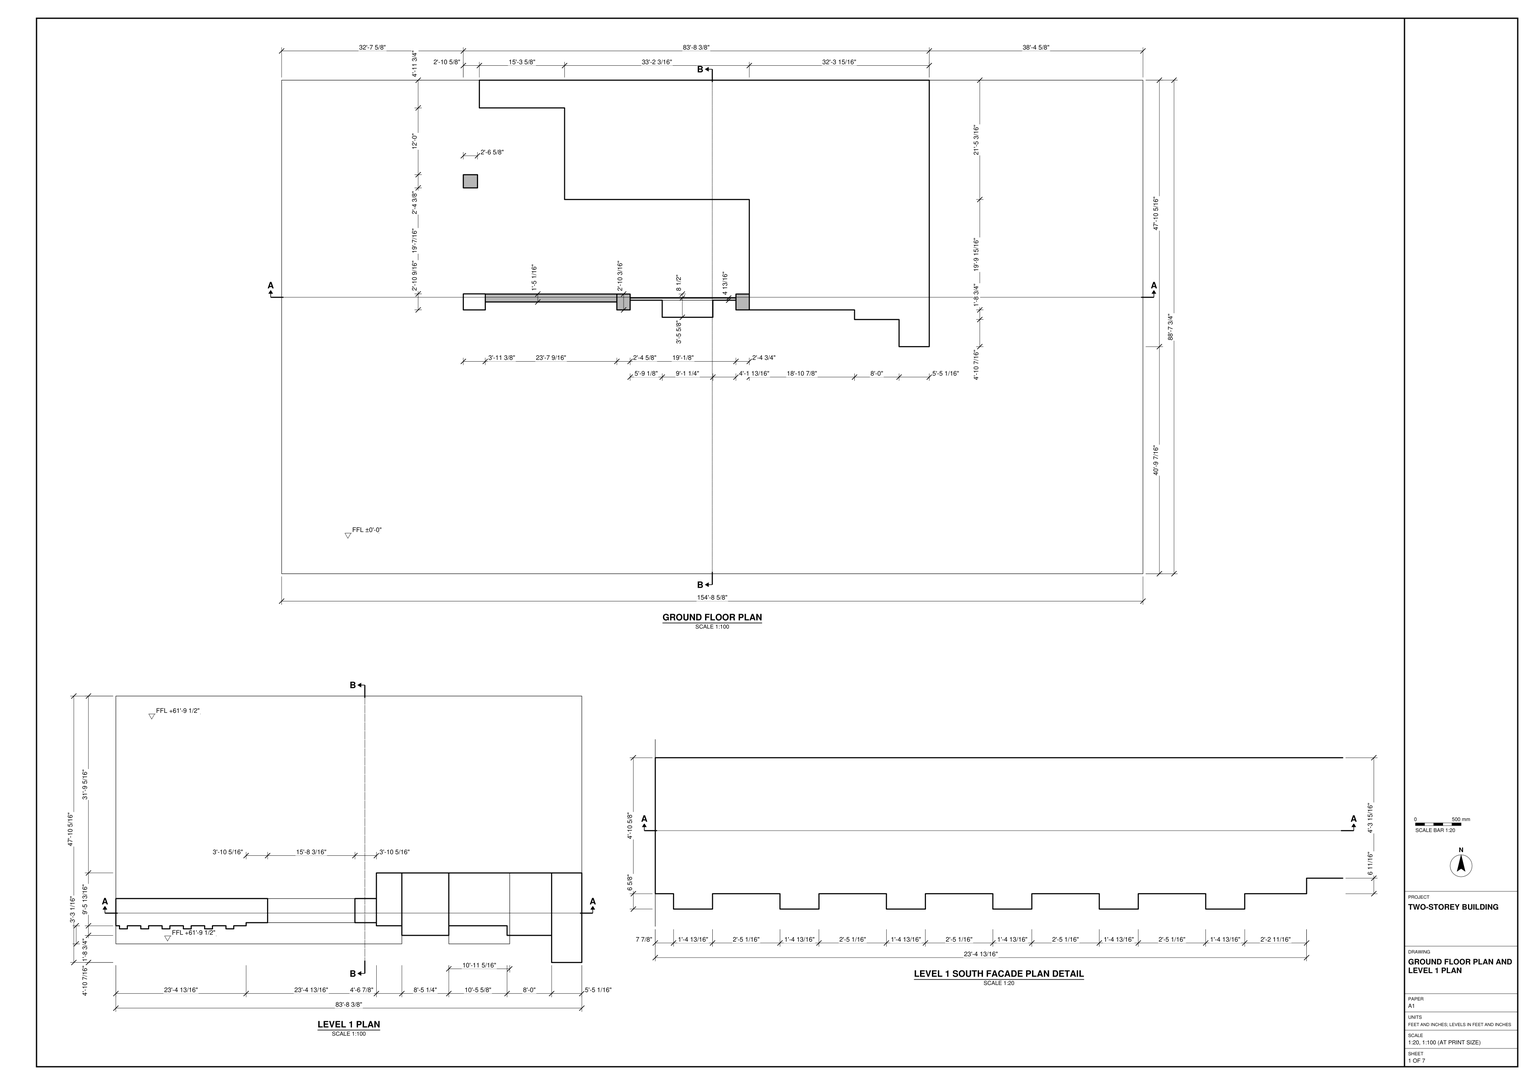
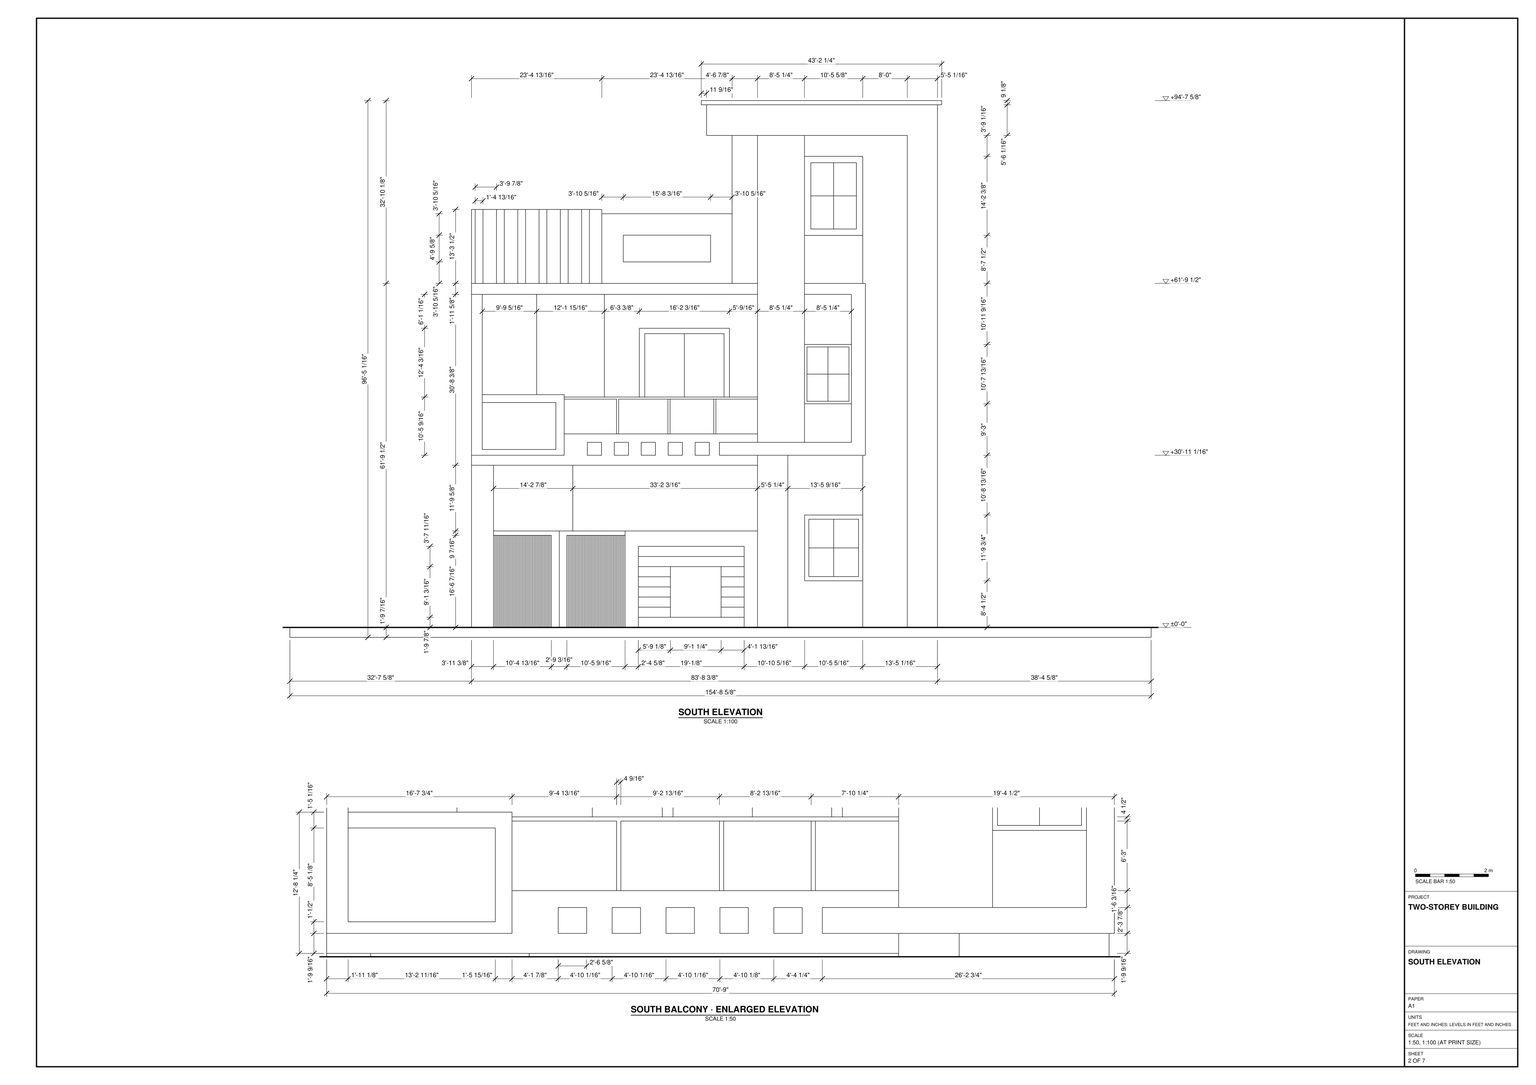
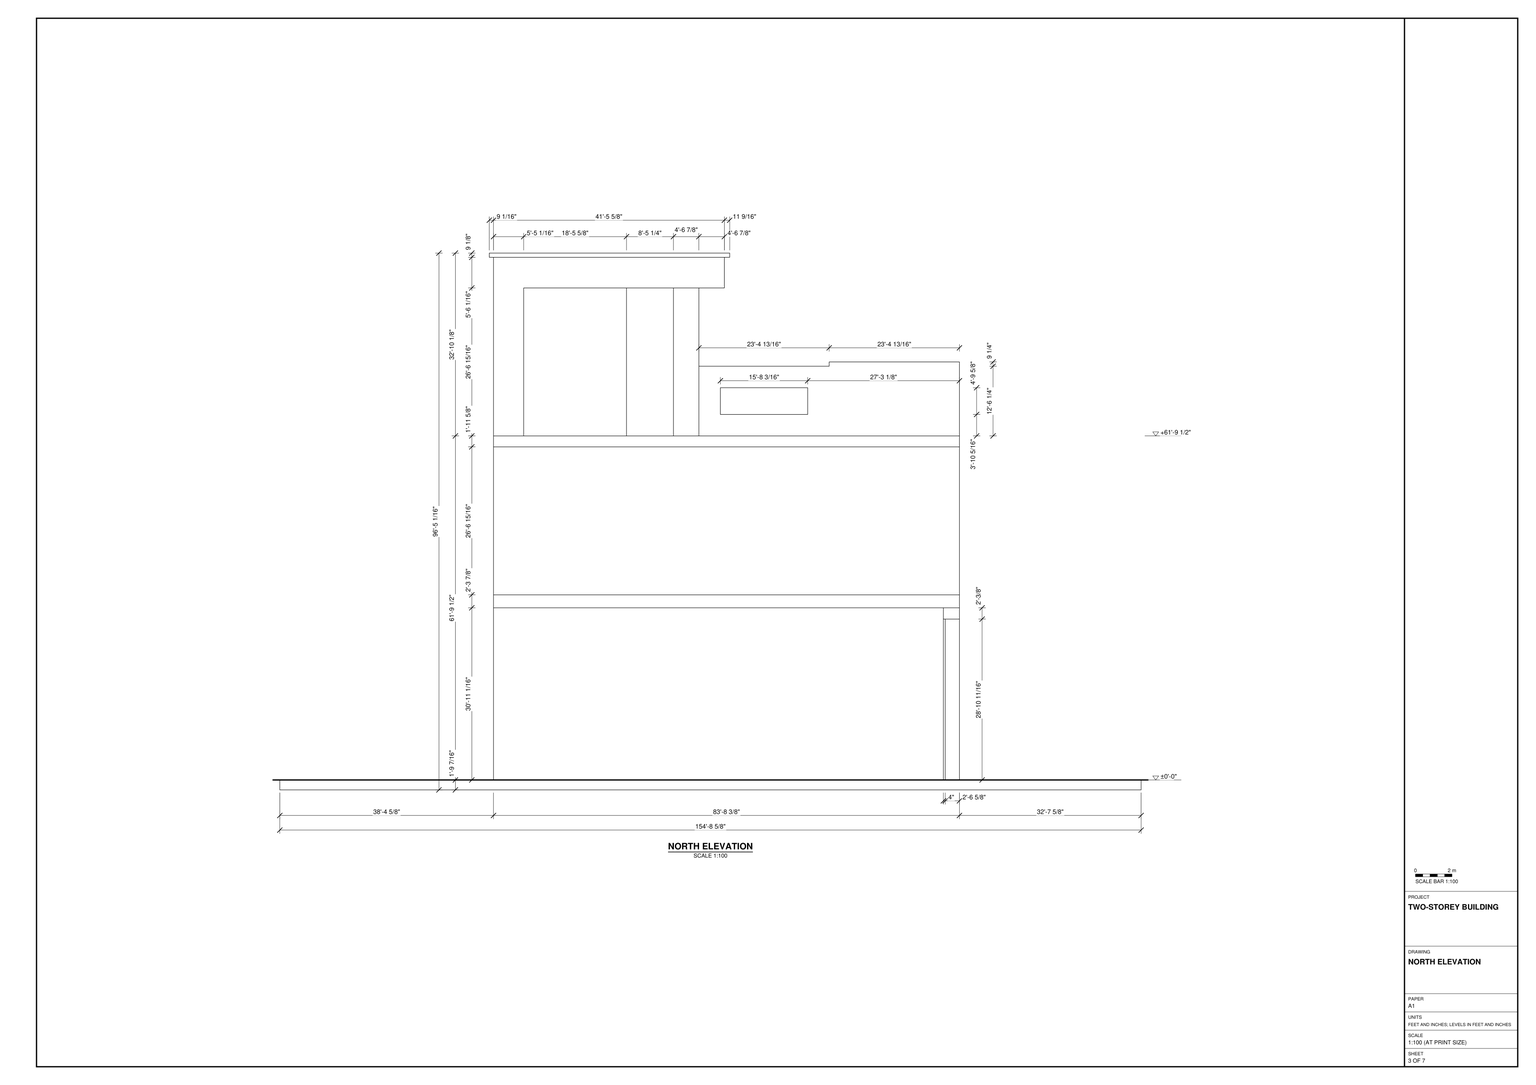
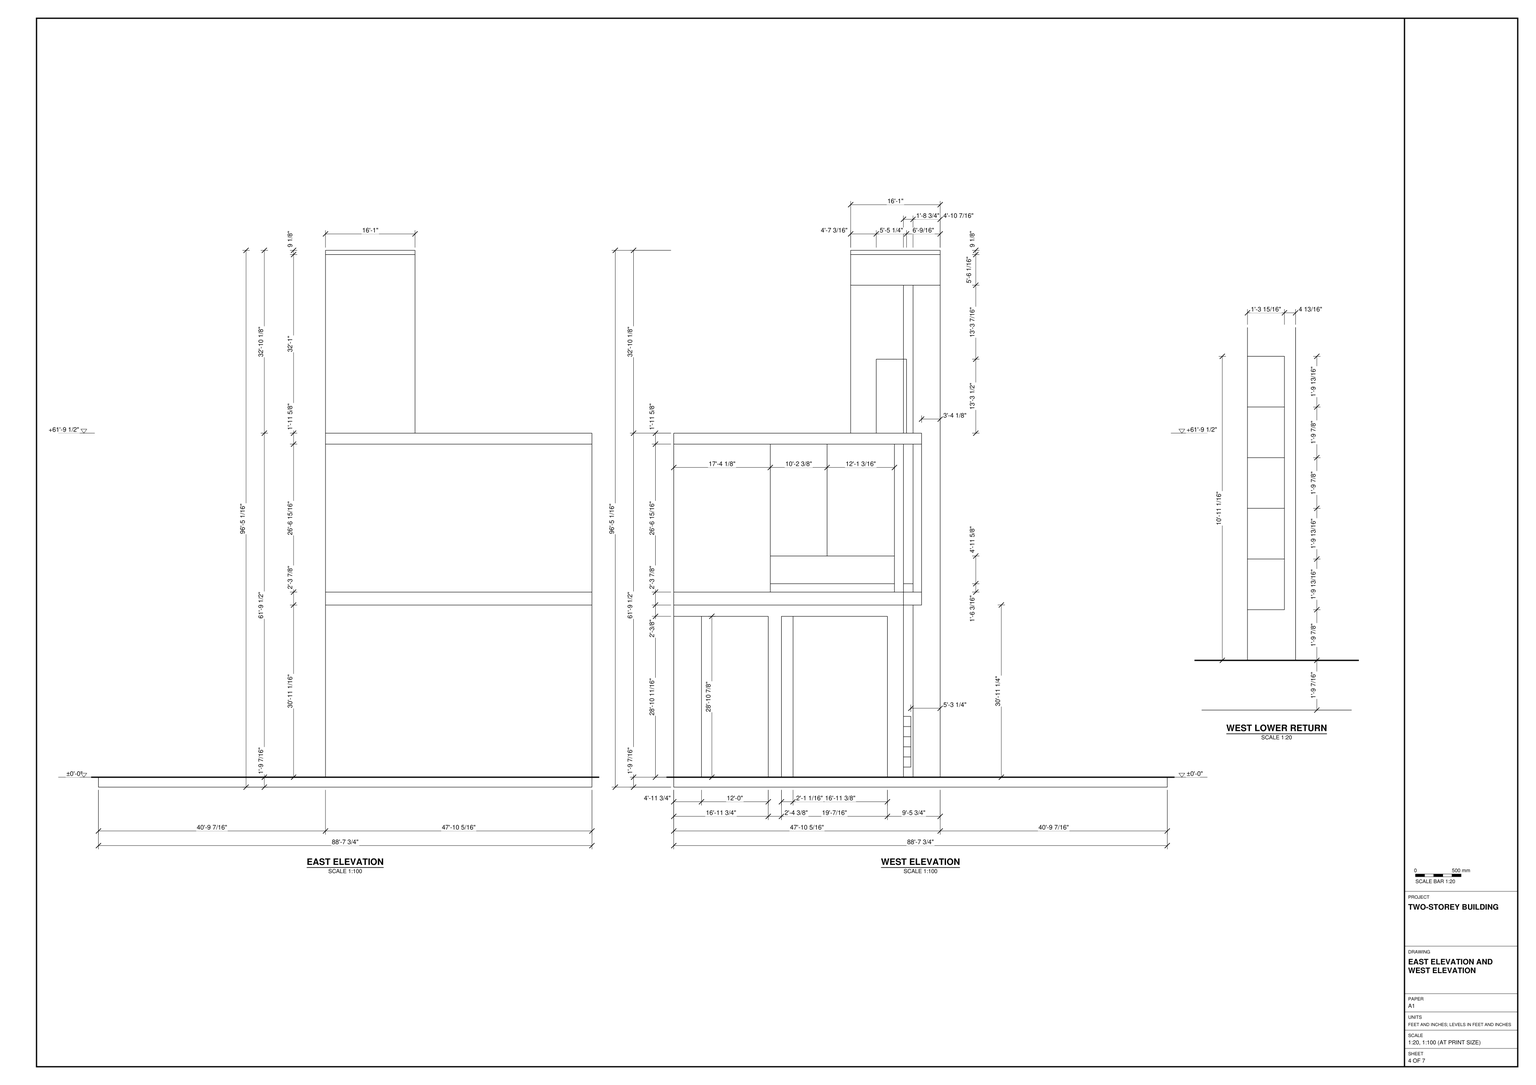
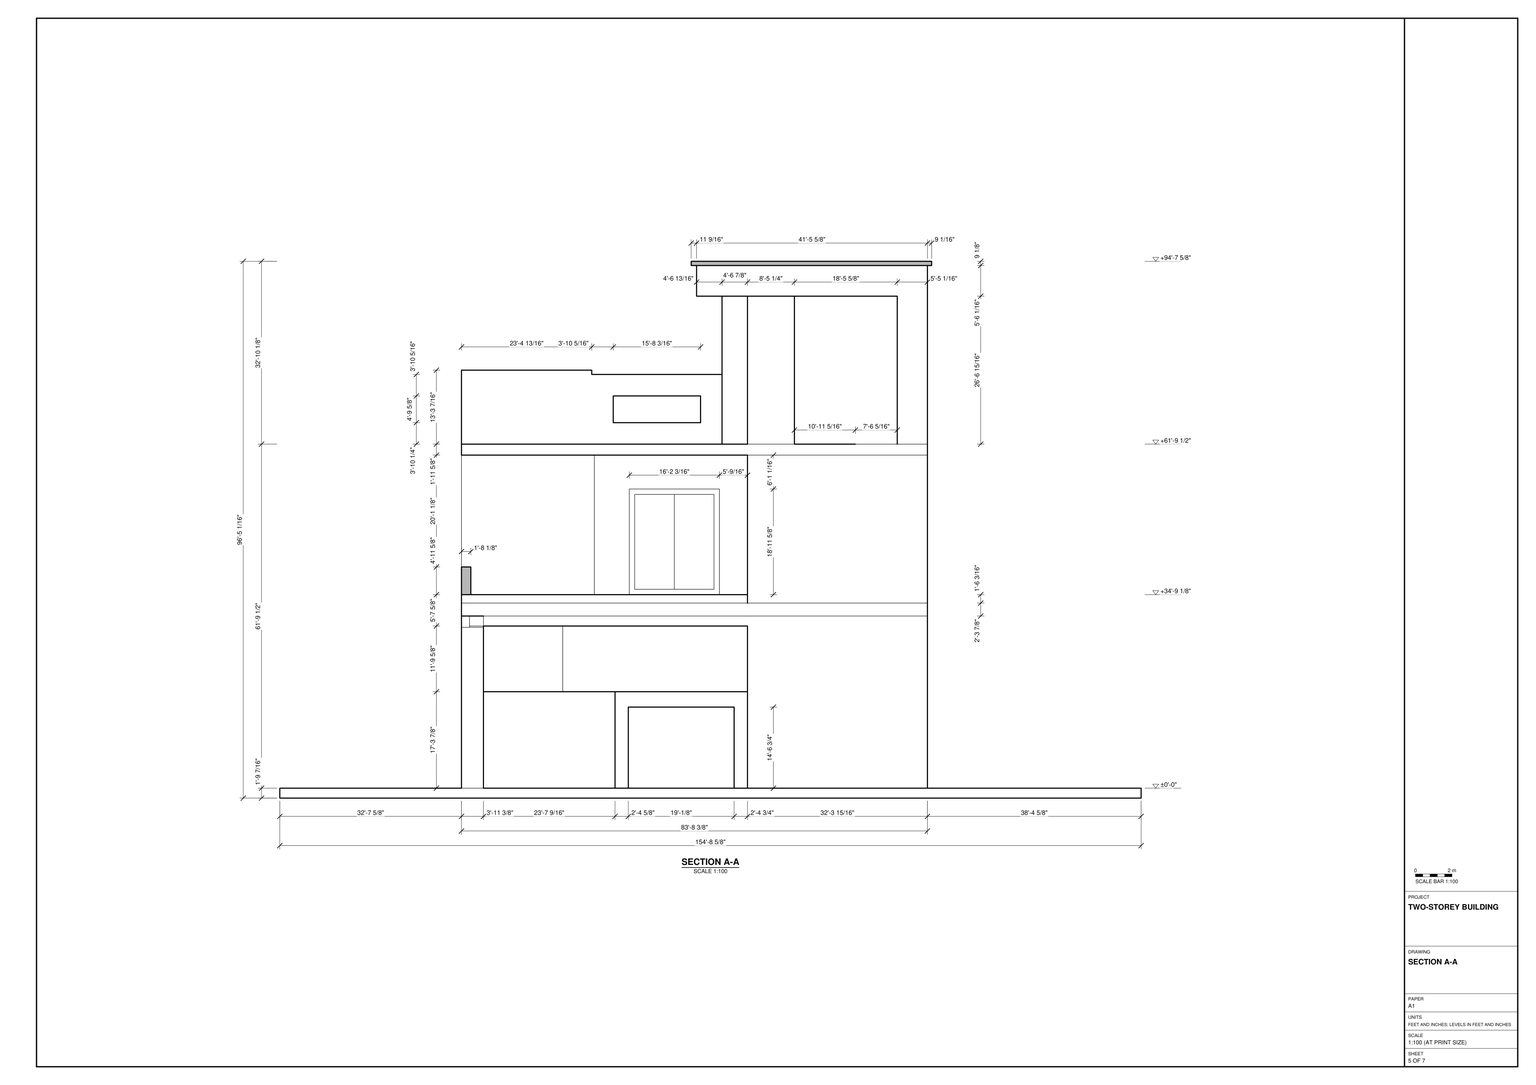
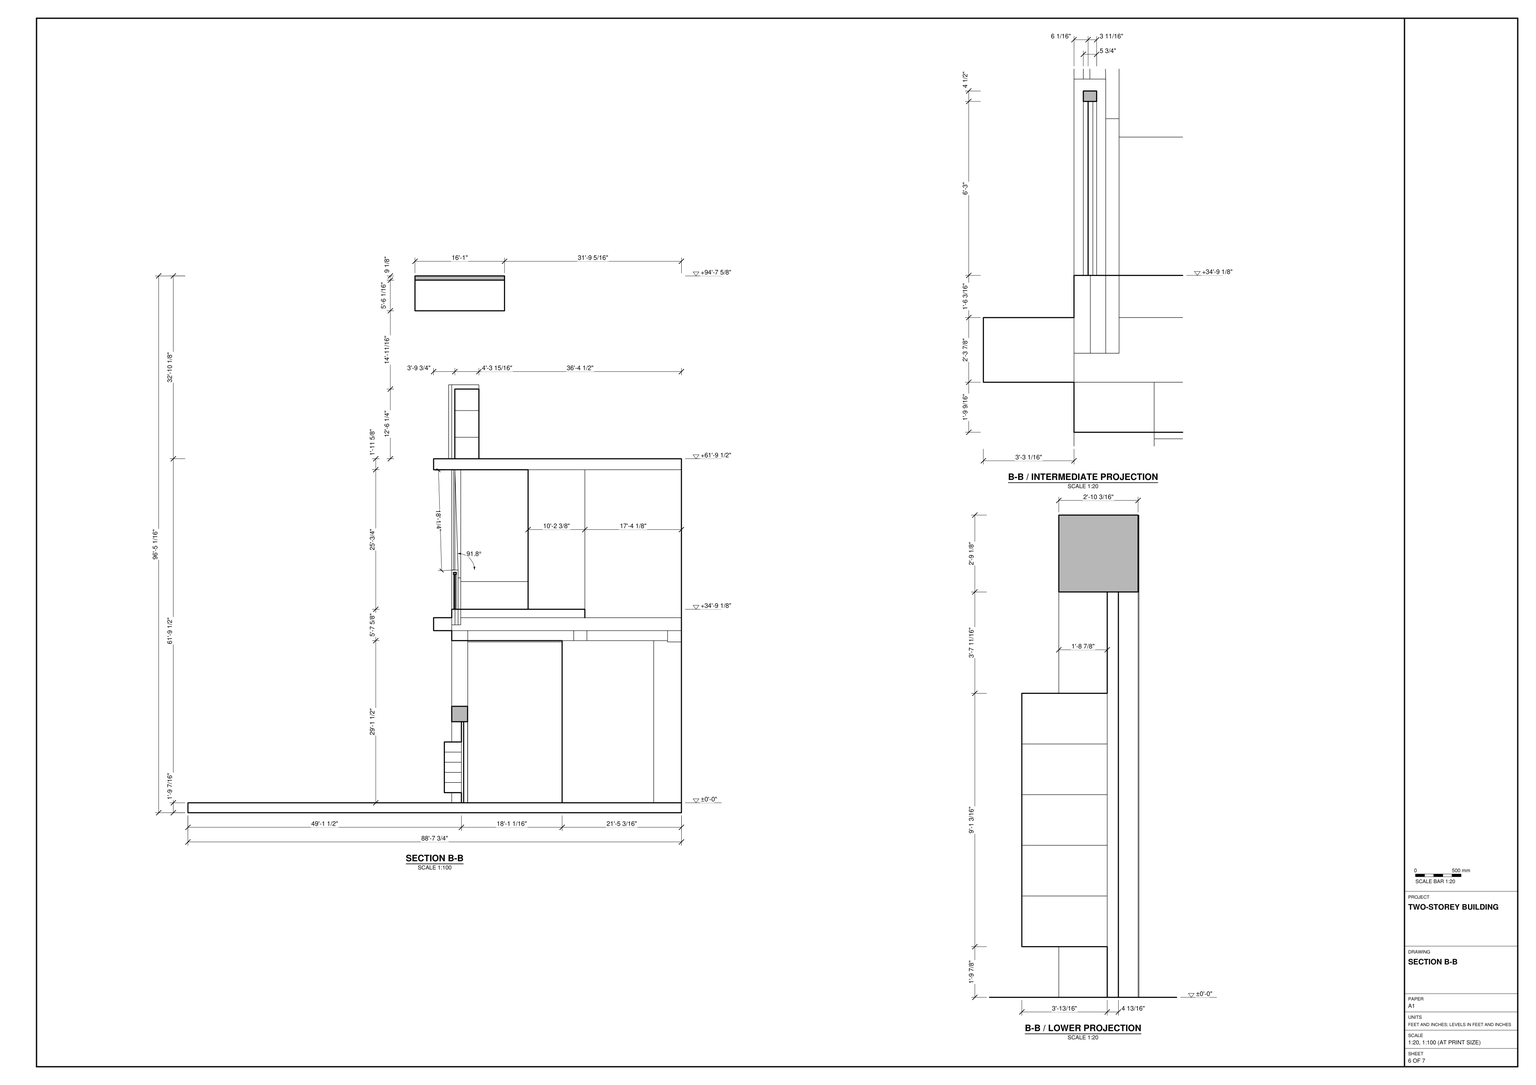
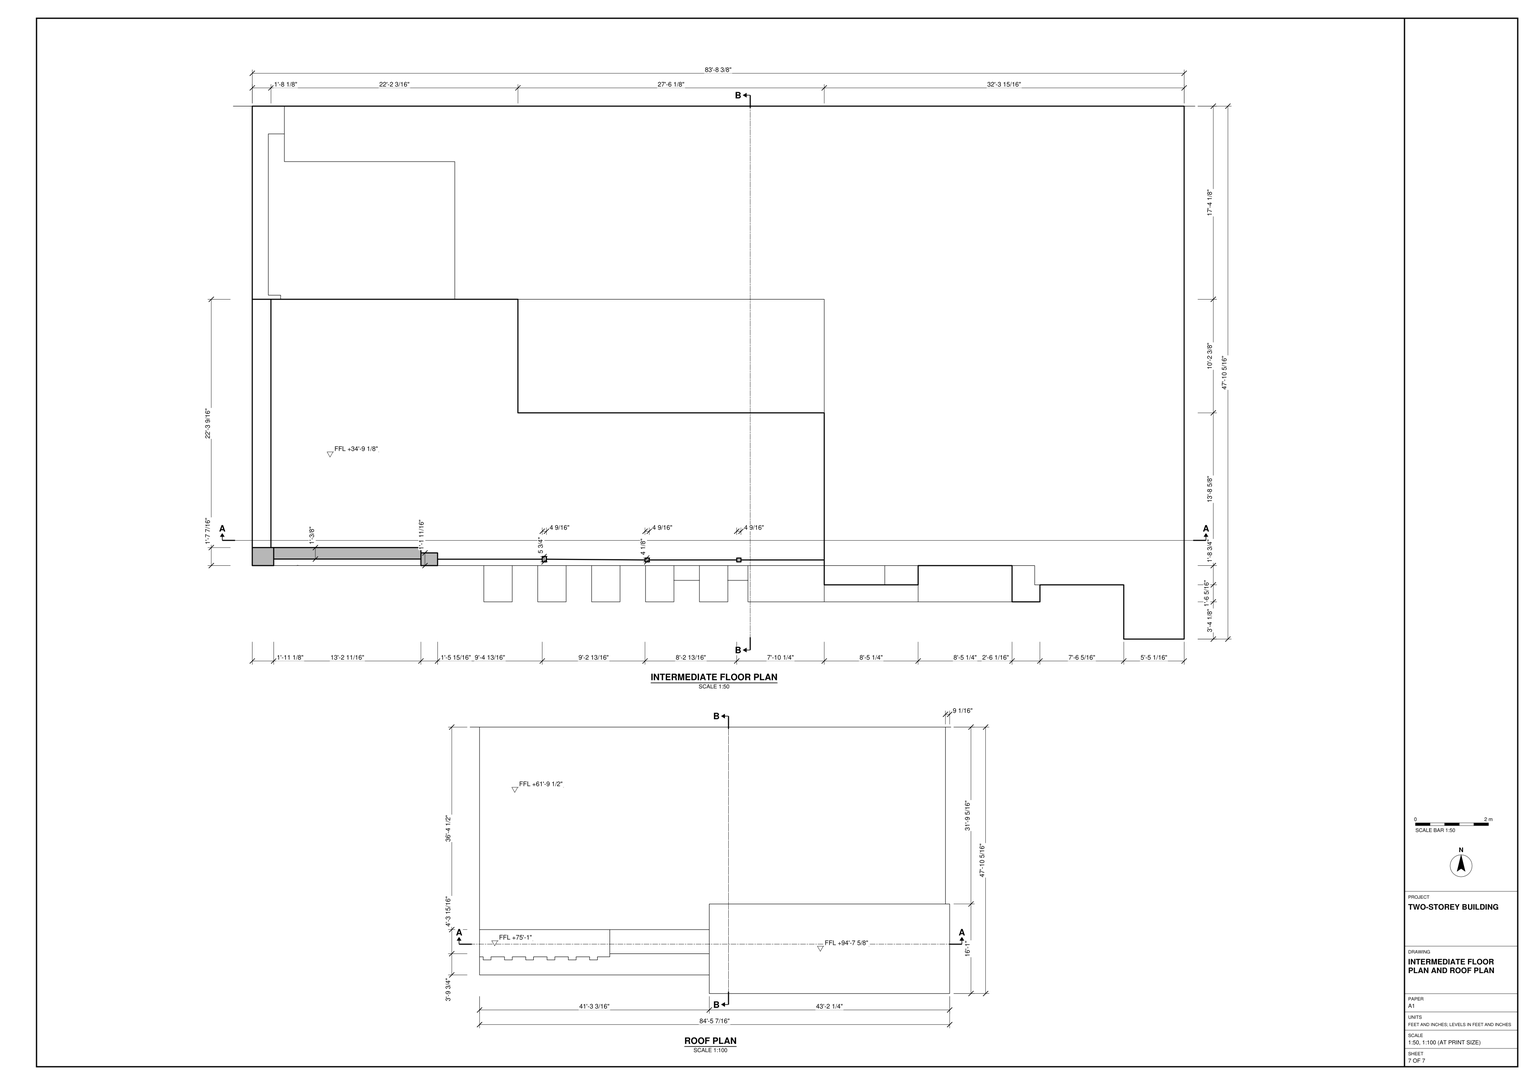
Build the two-storey building shown in task_files/diagram_01.pdf. Work in feet and inches. Including the rectangular ground slab, the model shall measure 154'-8 5/8" along X, 88'-7 3/4" along Y and 96'-5 1/16" in overall height. Set the ground floor at ±0'-0" and Level 1 at +61'-9 1/2".

Use the ground floor plan to position the building on the slab, leaving the broad open area to the south. Follow the stepped footprint and model the supports, walls and slabs at their drawn thicknesses. On the south face, place the ribbed panels and banded opening below the balcony. Use the enlarged balcony elevation to lay out the framed end panel, railing divisions and row of square details. Align the divided windows in the taller bay. Above Level 1, distinguish the low ribbed wall and its adjoining horizontal opening from the tall frame with its projecting roof cap. Include stairs, built-in joinery and main furniture only where the sheets show them.

Keep walls, slabs, roof elements and each furniture or joinery piece in separate groups or components, and use components for repeated parts. Decor and loose items may be any suitable library components. Save one SketchUp model as output_files/two_storey_building_with_a_projecting_south_balcony.skp.

# SketchUp Ruby script. Lengths in inches.
U = 1.inch
M = Sketchup.active_model
def pt(a) = Geom::Point3d.new(a.map { |v| v * U })
def face(e, loops, mat)
  f = e.add_face(loops[0].map { |a| pt(a) })
  loops[1..].each { |l| e.add_face(l.map { |a| pt(a) }).erase! }
  f.material = f.back_material = mat if mat
  f
end
# faces: each face lists its corners as indices into pts; further lists are holes
def faces(e, pts, list, mat = nil) = list.each { |f| face(e, (f[0].is_a?(Array) ? f : [f]).map { |l| l.map { |i| pts[i] } }, mat) }
# xy, xz, yz: faces in a plane at the given z, y or x. An outline is a flat list of corners, or four numbers for a rectangle; further outlines are holes
def ring(l) = l.size == 4 ? [[l[0], l[1]], [l[2], l[1]], [l[2], l[3]], [l[0], l[3]]] : l.each_slice(2).to_a
def flat(e, list, mat, &to3) = list.each { |f| face(e, (f[0].is_a?(Array) ? f : [f]).map { |l| ring(l).map { |u, v| to3.(u, v) } }, mat) }
def xy(e, z, list, mat = nil) = flat(e, list, mat) { |x, y| [x, y, z] }
def xz(e, y, list, mat = nil) = flat(e, list, mat) { |x, z| [x, y, z] }
def yz(e, x, list, mat = nil) = flat(e, list, mat) { |y, z| [x, y, z] }
def lines(e, pts, list) = list.each { |a, b| e.add_line(pt(pts[a]), pt(pts[b])) }
# prism: a flat outline (further loops are holes) pulled along v
def prism(e, loops, v, mat = nil)
  f = face(e, loops, mat); d = Geom::Vector3d.new(v.map { |x| x * U })
  f.pushpull(f.normal.samedirection?(d) ? d.length : -d.length)
end
def box(e, o, s, mat = nil) = prism(e, [[o, [o[0] + s[0], o[1], o[2]], [o[0] + s[0], o[1] + s[1], o[2]], [o[0], o[1] + s[1], o[2]]]], [0, 0, s[2]], mat)
def at(x, y, z, deg = 0) = Geom::Transformation.translation(pt([x, y, z])) * Geom::Transformation.rotation(ORIGIN, Z_AXIS, deg.degrees)
def axes(o, x, y, z) = Geom::Transformation.new([*x, 0, *y, 0, *z, 0, *pt(o).to_a, 1])
def part(name) = M.definitions.add(name)
# library, detail: a bought-in or finely detailed component or shape, given as its bounding box
def library(name, o, s) = part(name).tap { |d| box(d.entities, o, s) }
def detail(e, o, s) = box(e.add_group.entities, o, s)
def put(e, d, t, mat = nil) = e.add_instance(d, t).tap { |i| i.material = mat if mat }
def group(e, t, mat = nil) = e.add_group.tap { |g| g.transformation = t; g.material = mat if mat }.entities
root = M.entities
M.materials.add("[Blinds Roman Hobbled Blue]").color = [81, 82, 87]
M.materials.add("[Color M03]").color = [170, 170, 170]
M.materials.add("[Color M09]").color = [0, 0, 0]
M.materials.add("[Metal Panel]").color = [143, 157, 158]
M.materials.add("[Roofing Slate Tan]").color = [200, 175, 128]
M.materials.add("[Tile Travertine 2 inch]").color = [114, 112, 109]
M.materials.add("[Translucent Glass Blue]").color = [100, 149, 237]
M.materials["[Translucent Glass Blue]"].alpha = 0.5
M.materials.add("[Translucent Glass Gray]").color = [224, 224, 224]
M.materials["[Translucent Glass Gray]"].alpha = 0.5
xy(root,0,[[0,0,1856.625,1063.75]])
xy(root,21.4375,[[[0,0,1856.625,0,1856.625,1063.75,1396,1063.75,1396,489.4375,1330.9375,489.4375,1330.9375,547.875,1234.9375,547.875,1234.9375,568.625,979.34,568.625,979.34,589.5,751.22,589.5,751.22,568.625,722.59,568.625,722.59,585.72,439,585.72,439,568.625,391.625,568.625,391.625,603.1875,439,603.1875,439,602.8125,751.22,602.8125,751.22,594.3125,979.34,594.3125,979.34,602.8125,1008.09,602.8125,1008.09,806.5625,609.9,806.5625,609.9,1004,426.25,1004,426.25,1063.75,0,1063.75],[391.625,831.625,422.25,860.03]],[1330.9375,489.4375,1330.9375,547.875,1234.9375,547.875,1234.9375,568.625,1008.09,568.625,1008.09,806.5625,609.9,806.5625,609.9,1004,426.25,1004,426.25,1063.75,1396,1063.75,1396,489.4375],[722.59,568.625,751.22,602.8125],[979.34,568.625,1008.09,602.8125],[439,585.72,722.59,602.8125],
  [751.22,589.5,979.34,594.3125]])
xy(root,43.28,[[820.34,552.6875,929.56,589.5]])
xy(root,152.5,[[820.34,552.6875,929.56,589.5]])
xy(root,196.1875,[[751.22,568.625,784.47,589.5],[784.47,568.625,979.34,589.5],[751.22,589.5,784.47,594.3125],[784.47,589.5,979.34,594.3125],[751.22,594.3125,979.34,602.8125]])
xy(root,229.32,[[722.59,568.625,1008.09,602.8125],[439,585.72,722.59,602.8125]])
xy(root,368.125,[[391.625,603.1875,408.9375,831.625],[391.625,860.03,391.625,1063.75,426.25,1063.75,426.25,1033.875,408.9375,1033.875,408.9375,860.03]])
xy(root,370.9375,[[439,568.625,439,603.1875,408.9375,603.1875,408.9375,831.625,422.25,831.625,422.25,860.03,408.9375,860.03,408.9375,1033.875,426.25,1033.875,426.25,1004,609.9,1004,609.9,806.5625,1008.09,806.5625,1008.09,568.625]])
xy(root,392.5,[[641.21,529.5625,671.83,568.625],[699.3,529.5625,729.93,568.625],[757.4,529.5625,788.02,568.625],[815.49,529.5625,846.12,568.625],[873.59,529.5625,904.21,568.625],
  [925.86,529.5625,1008.09,568.625],[1008.09,529.5625,1073.37,568.625],[1073.37,529.5625,1073.37,568.625,1234.9375,568.625,1234.9375,547.875,1240.6,547.875,1240.6,529.5625],[391.625,568.625,439,568.625,439,603.1875,408.9375,603.1875,408.9375,831.625,422.25,831.625,422.25,860.03,408.9375,860.03,408.9375,1033.875,426.25,1033.875,426.25,1063.75,391.625,1063.75]])
xy(root,405,[[414.73,568.625,573.42,575.6875],[414.73,575.6875,573.42,582.3125],[414.73,582.3125,573.42,588.0625]])
xy(root,420.375,[[641.21,529.5625,671.83,568.625],[699.3,529.5625,729.93,568.625],[757.4,529.5625,788.02,568.625],[815.49,529.5625,846.12,568.625],[873.59,529.5625,904.21,568.625],
  [925.86,529.5625,1008.09,568.625],[1008.09,529.5625,1109.3125,547.875],[1109.3125,529.5625,1210.54,568.625]])
xy(root,438.5625,[[591.36,568.625,1008.09,568.625,1008.09,574.71,918.375,574.71,918.375,572.65,913.8125,572.65,913.8125,574.71,819.54,574.71,819.54,572.65,814.98,572.65,814.98,574.71,708.72,575.52,708.72,572.65,704.17,572.65,704.17,575.52,591.36,575.52],[814.98,572.65,819.54,576.77],[814.98,572.65,819.54,576.77],[913.8125,572.65,918.375,576.77],[913.8125,572.65,918.375,576.77],
  [814.98,574.71,814.98,576.77,819.54,576.77,819.54,574.71,913.8125,574.71,913.8125,576.77,918.375,576.77,918.375,574.71,1008.09,574.71,1008.09,733.25,677.94,733.25,677.94,855.625,411.75,855.625,411.75,588.0625,414.73,588.0625,414.73,582.3125,591.36,582.3125,591.36,575.52,704.17,575.52,704.17,578.4,708.72,578.4,708.72,575.52],[391.625,588.0625,411.75,855.625],[677.94,733.25,1008.09,855.625]])
xy(root,498.1875,[[391.625,588.0625,411.75,855.625]])
xy(root,506.125,[[414.73,568.625,425.91,575.6875],[425.91,568.625,439.79,575.6875],[439.79,568.625,573.42,575.6875],[414.73,575.6875,425.91,582.3125],[425.91,575.6875,439.79,582.3125],
  [439.79,575.6875,573.42,582.3125],[414.73,582.3125,425.91,588.0625],[425.91,582.3125,439.79,588.0625],[439.79,582.3125,573.42,588.0625]])
xy(root,513.5625,[[591.36,572.65,704.17,575.52],[708.72,572.65,708.72,575.52,814.98,574.71,814.98,572.65],[814.98,572.65,819.54,576.77],[819.54,572.65,913.8125,574.71],[913.8125,572.65,918.375,576.77],
  [918.375,572.65,1008.09,574.71],[814.98,574.71,708.72,575.52,708.72,578.4,1008.09,578.4,1008.09,575.52,918.375,574.71,918.375,576.77,913.8125,576.77,913.8125,574.71,819.54,574.71,819.54,576.77,814.98,576.77],[918.375,574.71,1008.09,575.52,1008.09,574.71],[591.36,575.52,704.17,578.4]])
xy(root,518.0625,[[591.36,572.65,1008.09,578.4]],"[Color M09]")
xy(root,523.19,[[414.73,568.625,591.36,568.625,591.36,582.3125,414.73,582.3125,414.73,575.47,532.02,575.47,532.02,572.66,414.73,572.66],[414.73,572.66,532.02,575.47]])
xy(root,739.3125,[[391.625,529.5625,414.73,568.625],[414.73,529.5625,414.73,572.66,532.02,572.66,532.02,575.47,414.73,575.47,414.73,588.0625,391.625,588.0625,391.625,855.625,677.94,855.625,677.94,733.25,1008.09,733.25,1008.09,529.5625],[1109.3125,529.5625,1210.54,568.625],[391.625,568.625,414.73,588.0625],[414.73,572.66,532.02,575.47]])
xy(root,762.9375,[[391.625,529.5625,1008.09,529.5625,1008.09,568.625,953.23,568.625,953.23,575.3125,672.43,575.3125,672.43,568.625,645.75,568.625,645.75,562,628.9375,562,628.9375,568.625,599.86,568.625,599.86,562,583.05,562,583.05,568.625,553.97,568.625,553.97,562,537.16,562,537.16,568.625,508.09,568.625,508.09,562,491.28,562,491.28,568.625,462.2,568.625,462.2,562,445.39,562,445.39,568.625,416.3125,568.625,416.3125,562,399.5,562,399.5,568.625,391.625,568.625],[1109.3125,529.5625,1240.6,529.5625,1240.6,547.875,1234.9375,547.875,1234.9375,568.625,1109.3125,568.625],[1234.9375,547.875,1240.6,547.875,1240.6,682.4375,1109.3125,682.4375,1109.3125,568.625,1234.9375,568.625],[399.5,562,416.3125,562,416.3125,568.625,445.39,568.625,445.39,562,462.2,562,462.2,568.625,491.28,568.625,491.28,562,508.09,562,508.09,568.625,537.16,568.625,537.16,562,553.97,562,553.97,568.625,583.05,568.625,583.05,562,599.86,562,599.86,568.625,628.9375,568.625,628.9375,562,645.75,562,645.75,568.625,672.43,568.625,672.43,575.3125,953.23,575.3125,953.23,627.25,391.625,627.25,391.625,568.625,399.5,568.625],[953.23,568.625,1008.09,682.4375],
  [391.625,627.25,953.23,627.25,953.23,682.4375,1396,682.4375,1396,1063.75,391.625,1063.75]])
xy(root,809.23,[[718.72,575.3125,906.9375,627.25]])
xy(root,866.43,[[1109.3125,568.625,1234.9375,582.6875]])
xy(root,866.86,[[718.72,575.3125,906.9375,627.25]])
xy(root,913.16,[[672.43,575.3125,953.23,627.25]])
xy(root,922.41,[[399.5,562,416.3125,562,416.3125,568.625,445.39,568.625,445.39,562,462.2,562,462.2,568.625,491.28,568.625,491.28,562,508.09,562,508.09,568.625,537.16,568.625,537.16,562,553.97,562,553.97,568.625,583.05,568.625,583.05,562,599.86,562,599.86,568.625,628.9375,568.625,628.9375,562,645.75,562,645.75,568.625,672.43,568.625,672.43,627.25,391.625,627.25,391.625,568.625,399.5,568.625]])
xy(root,1036.8,[[1109.3125,547.875,1234.9375,582.6875]])
xy(root,1081.875,[[898.375,489.4375,898.375,682.4375,953.23,682.4375,953.23,568.625,1008.09,568.625,1008.09,547.875,1330.9375,547.875,1330.9375,489.4375],[1008.09,547.875,1109.3125,682.4375],[1109.3125,547.875,1330.9375,682.4375],[953.23,568.625,1008.09,682.4375]])
xy(root,1147.9375,[[886.8125,489.4375,898.375,682.4375],[898.375,489.4375,1396,682.4375],[1396,489.4375,1405.0625,682.4375]])
xy(root,1157.0625,[[886.8125,489.4375,1405.0625,682.4375]])
xz(root,0,[[0,0,1856.625,21.4375]])
xz(root,489.4375,[[1330.9375,21.4375,1396,21.4375,1396,1147.9375,898.375,1147.9375,898.375,1081.875,1330.9375,1081.875],[886.8125,1147.9375,1405.0625,1157.0625]])
xz(root,529.5625,[[641.21,392.5,671.83,420.375],[699.3,392.5,729.93,420.375],[757.4,392.5,788.02,420.375],[815.49,392.5,846.12,420.375],[873.59,392.5,904.21,420.375],
  [925.86,392.5,1240.6,392.5,1240.6,762.9375,1109.3125,762.9375,1109.3125,739.3125,1210.54,739.3125,1210.54,420.375,925.86,420.375],[391.625,739.3125,1008.09,762.9375]])
xz(root,547.875,[[1234.9375,21.4375,1330.9375,21.4375,1330.9375,1081.875,1109.3125,1081.875,1109.3125,1036.8,1234.9375,1036.8,1234.9375,762.9375,1240.6,762.9375,1240.6,392.5,1234.9375,392.5]],"[Roofing Slate Tan]")
xz(root,547.875,[[1008.09,420.375,1109.3125,1081.875]],"[Tile Travertine 2 inch]")
xz(root,552.6875,[[820.34,43.28,929.56,152.5]],"[Tile Travertine 2 inch]")
xz(root,562,[[399.5,762.9375,416.3125,922.41],[445.39,762.9375,462.2,922.41],[491.28,762.9375,508.09,922.41],[537.16,762.9375,553.97,922.41],[583.05,762.9375,599.86,922.41],
  [628.9375,762.9375,645.75,922.41]],"[Color M03]")
xz(root,568.625,[[391.625,21.4375,439,370.9375],[722.59,21.4375,751.22,21.4375,751.22,196.1875,979.34,196.1875,979.34,21.4375,1008.09,21.4375,1008.09,229.32,722.59,229.32],[1073.37,21.4375,1234.9375,21.4375,1234.9375,121.94,1109.625,121.94,1109.625,263.69,1234.9375,263.69,1234.9375,392.5,1073.37,392.5],[391.625,392.5,591.36,392.5,591.36,523.19,414.73,523.19,414.73,506.125,573.42,506.125,573.42,405,414.73,405,414.73,739.3125,391.625,739.3125],[1109.3125,420.375,1210.54,503.52],
  [1109.3125,631.35,1210.54,739.3125],[391.625,762.9375,399.5,922.41],[416.3125,762.9375,445.39,922.41],[462.2,762.9375,491.28,922.41],[508.09,762.9375,537.16,922.41],
  [553.97,762.9375,583.05,922.41],[599.86,762.9375,628.9375,922.41],[645.75,762.9375,672.43,922.41],[953.23,762.9375,1008.09,1081.875],[1109.3125,762.9375,1234.9375,866.43]])
xz(root,568.625,[[1008.09,21.4375,1073.37,392.5],[[391.625,370.9375,1008.09,370.9375,1008.09,392.5,925.86,392.5,925.86,420.375,1008.09,420.375,1008.09,438.5625,591.36,438.5625,591.36,392.5,391.625,392.5],[815.49,392.5,846.12,420.375],[699.3,392.5,729.93,420.375],[641.21,392.5,671.83,420.375],[757.4,392.5,788.02,420.375],[873.59,392.5,904.21,420.375]]],"[Color M03]")
xz(root,568.625,[[[1109.625,121.94,1234.9375,263.69],[1118.7,131.01,1225.87,254.62]],[[1109.3125,503.52,1210.54,631.35],[1114.67,508.88,1205.18,625.99]]],"[Color M09]")
xz(root,568.625,[[1118.7,131.01,1172.28,192.82],[1172.28,131.01,1225.87,192.82],[1118.7,192.82,1172.28,254.62],[1172.28,192.82,1225.87,254.62],[1114.67,508.88,1159.92,567.43],
  [1159.92,508.88,1205.18,567.43],[1114.67,567.43,1159.92,625.99],[1159.92,567.43,1205.18,625.99]],"[Translucent Glass Blue]")
xz(root,572.65,[[704.17,438.5625,708.72,438.5625,708.72,513.5625,1008.09,513.5625,1008.09,518.0625,591.36,518.0625,591.36,513.5625,704.17,513.5625],[814.98,438.5625,819.54,513.5625],[913.8125,438.5625,918.375,513.5625]],"[Color M09]")
xz(root,572.66,[[414.73,523.19,532.02,739.3125]],"[Blinds Roman Hobbled Blue]")
xz(root,574.71,[[819.54,438.5625,913.8125,513.5625],[918.375,438.5625,1008.09,513.5625]],"[Translucent Glass Blue]")
xz(root,575.3125,[[[672.43,762.9375,953.23,913.16],[718.72,809.23,906.9375,866.86]]],"[Color M03]")
xz(root,575.47,[[414.73,523.19,532.02,739.3125]])
xz(root,575.52,[[591.36,438.5625,704.17,513.5625]],"[Translucent Glass Blue]")
xz(root,575.6875,[[414.73,405,573.42,506.125]],"[Tile Travertine 2 inch]")
xz(root,576.77,[[814.98,438.5625,819.54,513.5625],[913.8125,438.5625,918.375,513.5625]])
xz(root,578.4,[[704.17,438.5625,704.17,513.5625,591.36,513.5625,591.36,518.0625,1008.09,518.0625,1008.09,513.5625,708.72,513.5625,708.72,438.5625]])
xz(root,582.3125,[[414.73,405,573.42,420.375],[414.73,420.375,573.42,438.5625],[573.42,438.5625,573.42,506.125,414.73,506.125,414.73,523.19,591.36,523.19,591.36,438.5625]])
xz(root,582.6875,[[[1109.3125,866.43,1234.9375,1036.8],[1123.05,880.16,1221.2,1023.07]]],"[Color M09]")
xz(root,582.6875,[[1123.05,880.16,1172.125,951.62],[1172.125,880.16,1221.2,951.62],[1123.05,951.62,1172.125,1023.07],[1172.125,951.62,1221.2,1023.07]],"[Translucent Glass Blue]")
xz(root,585.72,[[597.02,21.4375,600.16,219.875],[600.16,21.4375,603.3,219.875],[603.3,21.4375,606.4375,219.875],[606.4375,21.4375,609.58,219.875],[609.58,21.4375,612.72,219.875],
  [612.72,21.4375,615.86,219.875],[615.86,21.4375,619,219.875],[619,21.4375,622.13,219.875],[622.13,21.4375,625.27,219.875],[625.27,21.4375,628.41,219.875],
  [628.41,21.4375,631.55,219.875],[631.55,21.4375,634.69,219.875],[634.69,21.4375,637.83,219.875],[637.83,21.4375,640.97,219.875],[640.97,21.4375,644.11,219.875],
  [644.11,21.4375,647.25,219.875],[647.25,21.4375,650.39,219.875],[650.39,21.4375,653.53,219.875],[653.53,21.4375,656.67,219.875],[656.67,21.4375,659.81,219.875],
  [659.81,21.4375,662.94,219.875],[662.94,21.4375,666.08,219.875],[666.08,21.4375,669.22,219.875],[669.22,21.4375,672.36,219.875],[672.36,21.4375,675.5,219.875],
  [675.5,21.4375,678.64,219.875],[678.64,21.4375,681.78,219.875],[681.78,21.4375,684.92,219.875],[684.92,21.4375,688.06,219.875],[688.06,21.4375,691.2,219.875],
  [691.2,21.4375,694.34,219.875],[694.34,21.4375,697.48,219.875],[697.48,21.4375,700.62,219.875],[700.62,21.4375,703.76,219.875],[703.76,21.4375,706.89,219.875],
  [706.89,21.4375,710.03,219.875],[710.03,21.4375,713.17,219.875],[713.17,21.4375,716.3125,219.875],[716.3125,21.4375,719.45,219.875],[719.45,21.4375,722.59,219.875]])
xz(root,585.72,[[439,21.4375,580.8,229.32],[580.8,21.4375,597.02,21.4375,597.02,219.875,722.59,219.875,722.59,229.32,580.8,229.32]],"[Metal Panel]")
xz(root,588.0625,[[414.73,405,573.42,506.125],[391.625,420.375,414.73,438.5625],[391.625,438.5625,411.75,498.1875],[411.75,438.5625,411.75,498.1875,391.625,498.1875,391.625,739.3125,414.73,739.3125,414.73,438.5625]])
xz(root,589.5,[[751.22,21.4375,979.34,43.28],[751.22,43.28,820.34,65.125],[929.56,43.28,979.34,65.125],[751.22,65.125,820.34,86.97],[929.56,65.125,979.34,86.97],
  [751.22,86.97,820.34,108.8125],[929.56,86.97,979.34,108.8125],[751.22,108.8125,820.34,130.66],[929.56,108.8125,979.34,130.66],[751.22,130.66,820.34,152.5],
  [929.56,130.66,979.34,152.5],[751.22,152.5,979.34,174.34],[751.22,174.34,979.34,196.1875]])
xz(root,594.3125,[[751.22,21.4375,979.34,196.1875]])
xz(root,602.8125,[[439,21.4375,722.59,229.32],[722.59,21.4375,722.59,229.32,1008.09,229.32,1008.09,21.4375,979.34,21.4375,979.34,196.1875,751.22,196.1875,751.22,21.4375]])
xz(root,603.1875,[[391.625,21.4375,439,368.125],[408.9375,368.125,439,370.9375],[408.9375,370.9375,439,392.5]])
xz(root,627.25,[[[391.625,762.9375,391.625,922.41,672.43,922.41,672.43,913.16,953.23,913.16,953.23,762.9375],[718.72,809.23,906.9375,866.86]]])
xz(root,682.4375,[[1330.9375,762.9375,1330.9375,1081.875,898.375,1081.875,898.375,1147.9375,1396,1147.9375,1396,762.9375],[953.23,762.9375,1008.09,1081.875],[1008.09,762.9375,1109.3125,1081.875],[1109.3125,762.9375,1330.9375,1081.875],[886.8125,1147.9375,1405.0625,1157.0625]])
xz(root,733.25,[[677.94,438.5625,753.34,438.5625,753.34,666.22,947.52,666.22,947.52,438.5625,1008.09,438.5625,1008.09,739.3125,677.94,739.3125]])
xz(root,733.25,[[[753.34,438.5625,947.52,666.22],[764.93,450.15,935.93,654.63]]],"[Color M09]")
xz(root,733.25,[[764.93,450.15,850.43,654.63],[850.43,450.15,935.93,654.63]],"[Translucent Glass Gray]")
xz(root,806.5625,[[609.9,21.4375,1008.09,370.9375]])
xz(root,831.625,[[391.625,21.4375,422.25,21.4375,422.25,370.9375,408.9375,370.9375,408.9375,368.125,391.625,368.125],[408.9375,370.9375,422.25,392.5]])
xz(root,855.625,[[391.625,420.375,1008.09,438.5625],[391.625,438.5625,411.75,498.1875],[411.75,438.5625,677.94,438.5625,677.94,739.3125,391.625,739.3125,391.625,498.1875,411.75,498.1875]])
xz(root,860.03,[[391.625,21.4375,422.25,368.125],[408.9375,368.125,422.25,370.9375],[408.9375,370.9375,422.25,392.5]])
xz(root,1004,[[426.25,21.4375,609.9,370.9375]])
xz(root,1033.875,[[408.9375,368.125,426.25,370.9375],[408.9375,370.9375,426.25,392.5]])
xz(root,1063.75,[[0,0,1856.625,21.4375],[426.25,21.4375,1396,392.5],[391.625,368.125,426.25,392.5],[391.625,392.5,1396,420.375],[391.625,420.375,1396,739.3125],
  [391.625,739.3125,1396,762.9375]])
yz(root,0,[[0,0,1063.75,21.4375]])
yz(root,391.625,[[568.625,21.4375,568.625,392.5,1063.75,392.5,1063.75,368.125,860.03,368.125,860.03,21.4375,831.625,21.4375,831.625,368.125,603.1875,368.125,603.1875,21.4375],[568.625,392.5,1063.75,420.375],[568.625,420.375,588.0625,739.3125],[588.0625,420.375,855.625,438.5625],[855.625,420.375,1063.75,739.3125],
  [588.0625,438.5625,855.625,498.1875],[529.5625,739.3125,1063.75,762.9375],[568.625,762.9375,627.25,922.41]])
yz(root,399.5,[[562,762.9375,568.625,922.41]])
yz(root,408.9375,[[603.1875,368.125,831.625,370.9375],[860.03,368.125,1033.875,370.9375],[603.1875,370.9375,831.625,392.5],[860.03,370.9375,1033.875,392.5]])
yz(root,411.75,[[588.0625,438.5625,855.625,498.1875]])
yz(root,414.73,[[568.625,405,575.6875,498.1875],[575.6875,405,582.3125,498.1875],[582.3125,405,588.0625,420.375],[582.3125,420.375,588.0625,438.5625],[582.3125,438.5625,588.0625,498.1875],
  [568.625,498.1875,575.6875,506.125],[575.6875,498.1875,582.3125,506.125],[582.3125,498.1875,588.0625,506.125],[568.625,506.125,582.3125,523.19],[582.3125,506.125,588.0625,506.125,588.0625,739.3125,575.47,739.3125,582.3125,523.19],
  [568.625,523.19,572.66,739.3125],[572.66,523.19,572.66,739.3125,575.47,739.3125,582.3125,523.19]])
yz(root,416.3125,[[562,762.9375,568.625,922.41]])
yz(root,422.25,[[831.625,21.4375,860.03,370.9375],[831.625,370.9375,860.03,392.5]])
yz(root,426.25,[[1004,21.4375,1004,370.9375,1033.875,370.9375,1033.875,368.125,1063.75,368.125,1063.75,21.4375],[1033.875,368.125,1063.75,392.5]])
yz(root,439,[[568.625,21.4375,585.72,21.4375,585.72,229.32,602.8125,229.32,602.8125,21.4375,603.1875,21.4375,603.1875,370.9375,568.625,370.9375],[585.72,21.4375,602.8125,229.32]])
yz(root,445.39,[[562,762.9375,568.625,922.41]])
yz(root,462.2,[[562,762.9375,568.625,922.41]])
yz(root,491.28,[[562,762.9375,568.625,922.41]])
yz(root,508.09,[[562,762.9375,568.625,922.41]])
yz(root,532.02,[[572.66,523.19,575.47,739.3125]])
yz(root,537.16,[[562,762.9375,568.625,922.41]])
yz(root,553.97,[[562,762.9375,568.625,922.41]])
yz(root,573.42,[[568.625,405,575.6875,506.125],[575.6875,405,582.3125,506.125],[582.3125,405,588.0625,506.125]])
yz(root,583.05,[[562,762.9375,568.625,922.41]])
yz(root,591.36,[[568.625,438.5625,575.52,438.5625,575.52,513.5625,572.65,513.5625,572.65,518.0625,578.4,518.0625,578.4,513.5625,575.52,513.5625,575.52,438.5625,582.3125,438.5625,582.3125,523.19,568.625,523.19]])
yz(root,599.86,[[562,762.9375,568.625,922.41]])
yz(root,609.9,[[806.5625,21.4375,1004,370.9375]])
yz(root,628.9375,[[562,762.9375,568.625,922.41]])
yz(root,641.21,[[529.5625,392.5,568.625,420.375]])
yz(root,645.75,[[562,762.9375,568.625,922.41]])
yz(root,671.83,[[529.5625,392.5,568.625,420.375]])
yz(root,672.43,[[568.625,762.9375,575.3125,762.9375,575.3125,913.16,627.25,913.16,627.25,922.41,568.625,922.41]])
yz(root,677.94,[[733.25,438.5625,855.625,739.3125]])
yz(root,699.3,[[529.5625,392.5,568.625,420.375]])
yz(root,704.17,[[572.65,438.5625,575.52,513.5625],[575.52,438.5625,578.4,513.5625]])
yz(root,708.72,[[572.65,438.5625,575.52,513.5625],[575.52,438.5625,578.4,513.5625]])
yz(root,718.72,[[575.3125,809.23,627.25,866.86]])
yz(root,722.59,[[568.625,21.4375,585.72,229.32],[585.72,21.4375,602.8125,229.32]])
yz(root,729.93,[[529.5625,392.5,568.625,420.375]])
yz(root,751.22,[[568.625,21.4375,589.5,196.1875],[589.5,21.4375,594.3125,196.1875],[594.3125,21.4375,602.8125,196.1875]])
yz(root,757.4,[[529.5625,392.5,568.625,420.375]])
yz(root,788.02,[[529.5625,392.5,568.625,420.375]])
yz(root,814.98,[[572.65,438.5625,574.71,513.5625],[574.71,438.5625,576.77,513.5625]])
yz(root,815.49,[[529.5625,392.5,568.625,420.375]])
yz(root,819.54,[[572.65,438.5625,574.71,513.5625],[574.71,438.5625,576.77,513.5625]])
yz(root,820.34,[[552.6875,43.28,589.5,65.125],[552.6875,65.125,589.5,86.97],[552.6875,86.97,589.5,108.8125],[552.6875,108.8125,589.5,130.66],[552.6875,130.66,589.5,152.5]])
yz(root,846.12,[[529.5625,392.5,568.625,420.375]])
yz(root,873.59,[[529.5625,392.5,568.625,420.375]])
yz(root,886.8125,[[489.4375,1147.9375,682.4375,1157.0625]])
yz(root,898.375,[[489.4375,1081.875,682.4375,1147.9375]])
yz(root,904.21,[[529.5625,392.5,568.625,420.375]])
yz(root,906.9375,[[575.3125,809.23,627.25,866.86]])
yz(root,913.8125,[[572.65,438.5625,574.71,513.5625],[574.71,438.5625,576.77,513.5625]])
yz(root,918.375,[[572.65,438.5625,574.71,513.5625],[574.71,438.5625,576.77,513.5625]])
yz(root,925.86,[[529.5625,392.5,568.625,420.375]])
yz(root,929.56,[[552.6875,43.28,589.5,65.125],[552.6875,65.125,589.5,86.97],[552.6875,86.97,589.5,108.8125],[552.6875,108.8125,589.5,130.66],[552.6875,130.66,589.5,152.5]])
yz(root,953.23,[[568.625,762.9375,568.625,1081.875,682.4375,1081.875,682.4375,762.9375,627.25,762.9375,627.25,913.16,575.3125,913.16,575.3125,762.9375],[575.3125,762.9375,627.25,913.16]])
yz(root,979.34,[[568.625,21.4375,589.5,196.1875],[589.5,21.4375,594.3125,196.1875],[594.3125,21.4375,602.8125,196.1875]])
yz(root,1008.09,[[568.625,21.4375,602.8125,229.32],[602.8125,21.4375,602.8125,229.32,568.625,229.32,568.625,370.9375,806.5625,370.9375,806.5625,21.4375],[547.875,420.375,568.625,438.5625],[568.625,420.375,855.625,438.5625],[547.875,438.5625,547.875,739.3125,733.25,739.3125,733.25,438.5625,574.71,438.5625,574.71,513.5625,578.4,513.5625,578.4,518.0625,572.65,518.0625,572.65,513.5625,574.71,513.5625,574.71,438.5625],
  [529.5625,739.3125,547.875,762.9375],[547.875,762.9375,568.625,1081.875],[568.625,762.9375,682.4375,1081.875]])
yz(root,1109.3125,[[547.875,420.375,568.625,739.3125],[529.5625,739.3125,547.875,762.9375],[547.875,762.9375,568.625,762.9375,568.625,866.43,582.6875,866.43,582.6875,1036.8,547.875,1036.8],[568.625,762.9375,568.625,866.43,582.6875,866.43,582.6875,1036.8,547.875,1036.8,547.875,1081.875,682.4375,1081.875,682.4375,762.9375]])
yz(root,1210.54,[[529.5625,420.375,568.625,739.3125]])
yz(root,1234.9375,[[547.875,21.4375,568.625,392.5],[547.875,762.9375,547.875,1036.8,582.6875,1036.8,582.6875,866.43,568.625,866.43,568.625,762.9375]])
yz(root,1240.6,[[529.5625,392.5,547.875,762.9375]])
yz(root,1330.9375,[[489.4375,21.4375,547.875,1081.875],[547.875,762.9375,682.4375,1081.875]])
yz(root,1396,[[489.4375,21.4375,1063.75,392.5],[489.4375,392.5,1063.75,420.375],[489.4375,420.375,1063.75,739.3125],[489.4375,739.3125,1063.75,762.9375],[489.4375,762.9375,682.4375,1147.9375]])
yz(root,1405.0625,[[489.4375,1147.9375,682.4375,1157.0625]])
yz(root,1856.625,[[0,0,1063.75,21.4375]])
p = [[814.98,574.71,513.5625],[708.72,575.52,513.5625],[708.72,575.52,438.5625],[814.98,574.71,438.5625],[563.8,585.72,21.4375],[563.8,585.72,219.875],
  [439,568.625,219.875],[560.68,585.72,21.4375],[560.68,585.72,219.875],[557.5625,585.72,21.4375],[557.5625,585.72,219.875],[554.44,585.72,21.4375],
  [554.44,585.72,219.875],[551.32,585.72,21.4375],[551.32,585.72,219.875],[548.2,585.72,21.4375],[548.2,585.72,219.875],[545.08,585.72,21.4375],
  [545.08,585.72,219.875],[541.96,585.72,21.4375],[541.96,585.72,219.875],[538.84,585.72,21.4375],[538.84,585.72,219.875],[535.72,585.72,21.4375],
  [535.72,585.72,219.875],[532.6,585.72,21.4375],[532.6,585.72,219.875],[529.48,585.72,21.4375],[529.48,585.72,219.875],[526.36,585.72,21.4375],
  [526.36,585.72,219.875],[523.24,585.72,21.4375],[523.24,585.72,219.875],[520.12,585.72,21.4375],[520.12,585.72,219.875],[517,585.72,21.4375],
  [517,585.72,219.875],[513.88,585.72,21.4375],[513.88,585.72,219.875],[510.76,585.72,21.4375],[510.76,585.72,219.875],[507.64,585.72,21.4375],
  [507.64,585.72,219.875],[504.52,585.72,21.4375],[504.52,585.72,219.875],[501.4,585.72,21.4375],[501.4,585.72,219.875],[498.28,585.72,21.4375],
  [498.28,585.72,219.875],[495.16,585.72,21.4375],[495.16,585.72,219.875],[492.04,585.72,21.4375],[492.04,585.72,219.875],[488.92,585.72,21.4375],
  [488.92,585.72,219.875],[485.8,585.72,21.4375],[485.8,585.72,219.875],[482.68,585.72,21.4375],[482.68,585.72,219.875],[479.5625,585.72,21.4375],
  [479.5625,585.72,219.875],[476.44,585.72,21.4375],[476.44,585.72,219.875],[473.32,585.72,21.4375],[473.32,585.72,219.875],[470.2,585.72,21.4375],
  [470.2,585.72,219.875],[467.08,585.72,21.4375],[467.08,585.72,219.875],[463.96,585.72,21.4375],[463.96,585.72,219.875],[460.84,585.72,21.4375],
  [460.84,585.72,219.875],[457.72,585.72,21.4375],[457.72,585.72,219.875],[454.6,585.72,21.4375],[454.6,585.72,219.875],[451.48,585.72,21.4375],
  [451.48,585.72,219.875],[448.36,585.72,21.4375],[448.36,585.72,219.875],[445.24,585.72,21.4375],[445.24,585.72,219.875],[442.12,585.72,21.4375],
  [442.12,585.72,219.875]]
faces(root,p,[[0,1,2,3]],"[Translucent Glass Blue]")
lines(root,p,[[4,5],[5,6],[7,8],[9,10],[11,12],[13,14],[15,16],[17,18],[19,20],[21,22],[23,24],[25,26],
  [27,28],[29,30],[31,32],[33,34],[35,36],[37,38],[39,40],[41,42],[43,44],[45,46],[47,48],[49,50],
  [51,52],[53,54],[55,56],[57,58],[59,60],[61,62],[63,64],[65,66],[67,68],[69,70],[71,72],[73,74],
  [75,76],[77,78],[79,80],[81,82],[83,84]])
